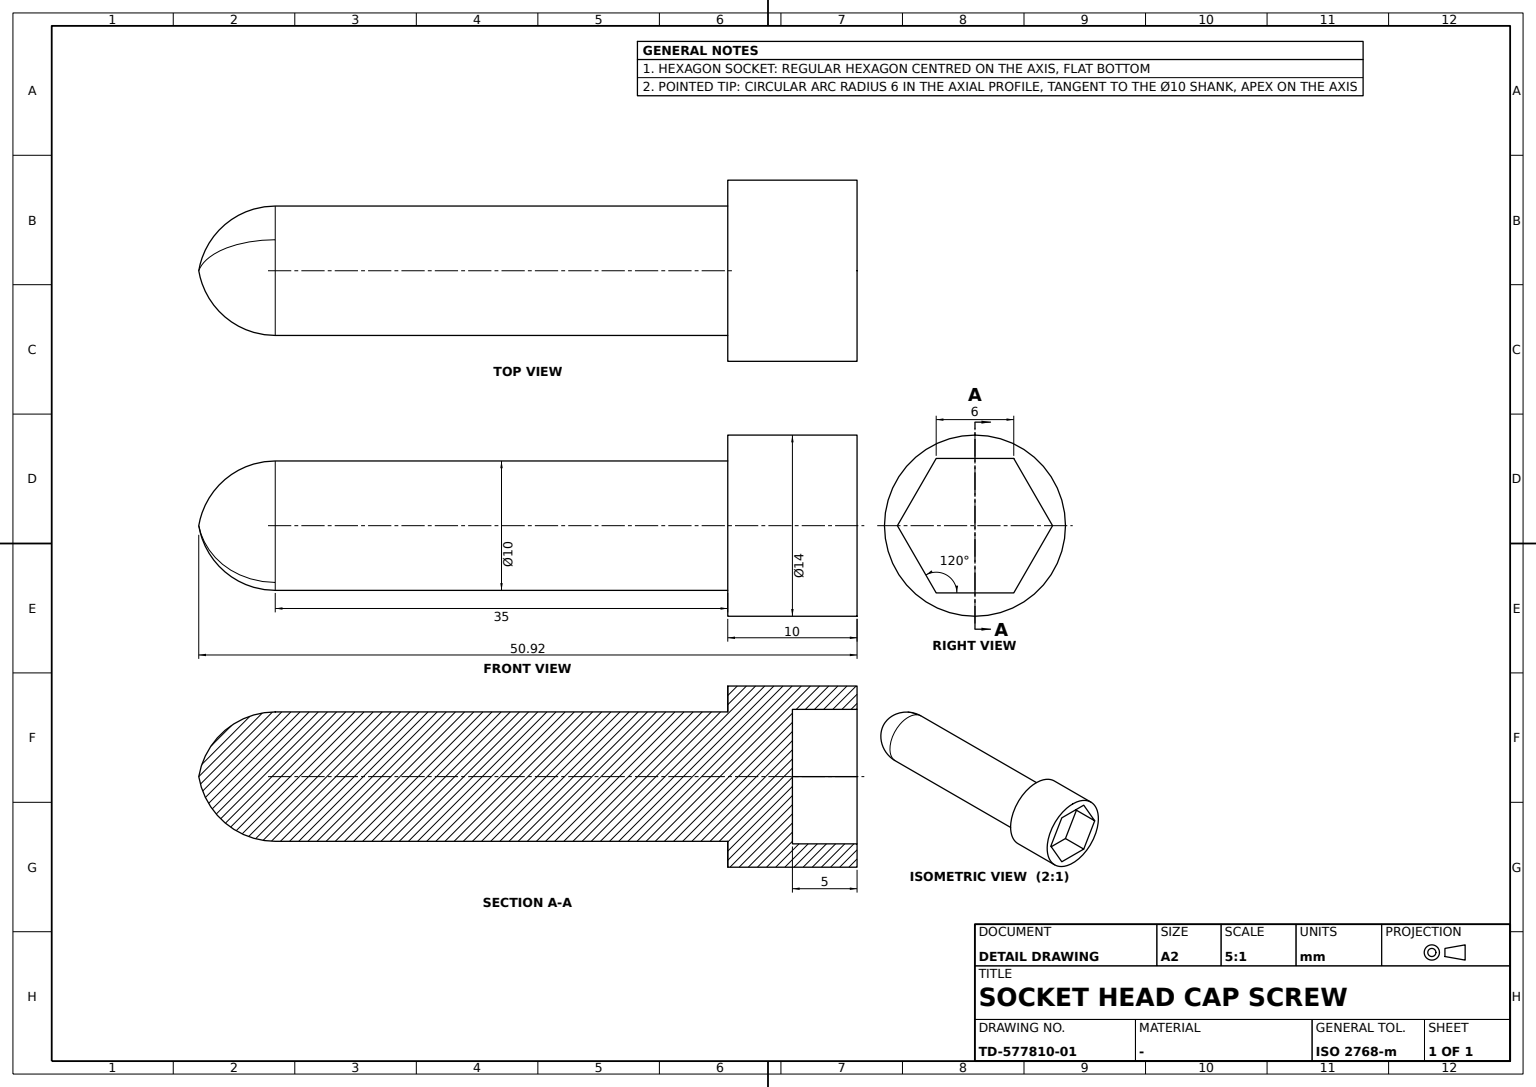
ISO-10303-21;
HEADER;
FILE_DESCRIPTION((''),'2;1');
FILE_NAME('','',(''),(''),'','','');
FILE_SCHEMA(('AUTOMOTIVE_DESIGN'));
ENDSEC;
DATA;
#1=APPLICATION_CONTEXT('');
#2=PRODUCT_CONTEXT('',#1,'mechanical');
#3=PRODUCT('','','',(#2));
#4=PRODUCT_DEFINITION_FORMATION('','',#3);
#5=PRODUCT_DEFINITION_CONTEXT('',#1,'design');
#6=PRODUCT_DEFINITION('','',#4,#5);
#7=PRODUCT_DEFINITION_SHAPE('','',#6);
#8=(LENGTH_UNIT()NAMED_UNIT(*)SI_UNIT(.MILLI.,.METRE.));
#9=(NAMED_UNIT(*)PLANE_ANGLE_UNIT()SI_UNIT($,.RADIAN.));
#10=(NAMED_UNIT(*)SI_UNIT($,.STERADIAN.)SOLID_ANGLE_UNIT());
#11=UNCERTAINTY_MEASURE_WITH_UNIT(LENGTH_MEASURE(0.005),#8,'distance_accuracy_value','');
#12=(GEOMETRIC_REPRESENTATION_CONTEXT(3)GLOBAL_UNCERTAINTY_ASSIGNED_CONTEXT((#11))GLOBAL_UNIT_ASSIGNED_CONTEXT((#8,#9,#10))REPRESENTATION_CONTEXT('',''));
#13=CARTESIAN_POINT('',(0.,-3.,-5.196152));
#14=VERTEX_POINT('',#13);
#15=CARTESIAN_POINT('',(0.,3.,-5.196152));
#16=VERTEX_POINT('',#15);
#17=CARTESIAN_POINT('',(0.,0.,-5.196152));
#18=DIRECTION('',(0.,1.,0.));
#19=VECTOR('',#18,1000.);
#20=LINE('',#17,#19);
#21=EDGE_CURVE('',#14,#16,#20,.T.);
#22=ORIENTED_EDGE('',*,*,#21,.T.);
#23=CARTESIAN_POINT('',(-5.,3.,-5.196152));
#24=VERTEX_POINT('',#23);
#25=DIRECTION('',(-1.,0.,0.));
#26=VECTOR('',#25,1000.);
#27=LINE('',#15,#26);
#28=EDGE_CURVE('',#16,#24,#27,.T.);
#29=ORIENTED_EDGE('',*,*,#28,.T.);
#30=CARTESIAN_POINT('',(-5.,-3.,-5.196152));
#31=VERTEX_POINT('',#30);
#32=LINE('',#30,#19);
#33=EDGE_CURVE('',#31,#24,#32,.T.);
#34=ORIENTED_EDGE('',*,*,#33,.F.);
#35=LINE('',#13,#26);
#36=EDGE_CURVE('',#14,#31,#35,.T.);
#37=ORIENTED_EDGE('',*,*,#36,.F.);
#38=EDGE_LOOP('',(#22,#29,#34,#37));
#39=FACE_BOUND('',#38,.T.);
#40=DIRECTION('',(0.,0.,1.));
#41=AXIS2_PLACEMENT_3D('',#13,#40,#18);
#42=PLANE('',#41);
#43=ADVANCED_FACE('',(#39),#42,.T.);
#44=CARTESIAN_POINT('',(-10.,0.,7.));
#45=VERTEX_POINT('',#44);
#46=CARTESIAN_POINT('',(-10.,0.,0.));
#47=AXIS2_PLACEMENT_3D('',#46,#25,#40);
#48=CIRCLE('',#47,7.);
#49=EDGE_CURVE('',#45,#45,#48,.T.);
#50=ORIENTED_EDGE('',*,*,#49,.F.);
#51=EDGE_LOOP('',(#50));
#52=FACE_BOUND('',#51,.T.);
#53=CARTESIAN_POINT('',(0.,0.,7.));
#54=VERTEX_POINT('',#53);
#55=CARTESIAN_POINT('',(0.,0.,0.));
#56=AXIS2_PLACEMENT_3D('',#55,#25,#40);
#57=CIRCLE('',#56,7.);
#58=EDGE_CURVE('',#54,#54,#57,.T.);
#59=ORIENTED_EDGE('',*,*,#58,.T.);
#60=EDGE_LOOP('',(#59));
#61=FACE_BOUND('',#60,.T.);
#62=CARTESIAN_POINT('',(-25.45804,0.,0.));
#63=AXIS2_PLACEMENT_3D('',#62,#25,#18);
#64=CYLINDRICAL_SURFACE('',#63,7.);
#65=ADVANCED_FACE('',(#52,#61),#64,.T.);
#66=CARTESIAN_POINT('',(-50.91608,0.,0.));
#67=VERTEX_POINT('',#66);
#68=CARTESIAN_POINT('',(-45.,-2.397128,-4.387913));
#69=VERTEX_POINT('',#68);
#70=CARTESIAN_POINT('',(-46.403166,-2.397,-4.38768));
#71=CARTESIAN_POINT('',(-49.203342,-1.904979,-3.487041));
#72=CARTESIAN_POINT('',(-50.681957,-0.663283,-1.214132));
#73=B_SPLINE_CURVE_WITH_KNOTS('',3,(#68,#70,#71,#72,#66),.UNSPECIFIED.,.F.,.F.,(4,1,4),(1.004688475,5.214733218,9.424777961),.UNSPECIFIED.);
#74=EDGE_CURVE('',#67,#69,#73,.F.);
#75=ORIENTED_EDGE('',*,*,#74,.F.);
#76=CARTESIAN_POINT('',(-45.,2.397128,4.387913));
#77=VERTEX_POINT('',#76);
#78=CARTESIAN_POINT('',(-50.681957,0.663283,1.214132));
#79=CARTESIAN_POINT('',(-49.203342,1.904979,3.487041));
#80=CARTESIAN_POINT('',(-46.403166,2.397,4.38768));
#81=B_SPLINE_CURVE_WITH_KNOTS('',3,(#66,#78,#79,#80,#76),.UNSPECIFIED.,.F.,.F.,(4,1,4),(1.004688475,5.214733218,9.424777961),.UNSPECIFIED.);
#82=EDGE_CURVE('',#67,#77,#81,.T.);
#83=ORIENTED_EDGE('',*,*,#82,.T.);
#84=CARTESIAN_POINT('',(-45.,-1.248375,-5.015479));
#85=CARTESIAN_POINT('',(-45.,1.558696,-5.316123));
#86=CARTESIAN_POINT('',(-45.,4.863313,-2.65684));
#87=CARTESIAN_POINT('',(-45.,5.31553,1.560716));
#88=CARTESIAN_POINT('',(-45.,3.545881,3.760346));
#89=B_SPLINE_CURVE_WITH_KNOTS('',3,(#68,#84,#85,#86,#87,#88,#76),.UNSPECIFIED.,.F.,.F.,(4,1,1,1,4),(26.061944902,29.988935719,33.915926536,37.842917353,41.76990817),.UNSPECIFIED.);
#90=EDGE_CURVE('',#77,#69,#89,.F.);
#91=ORIENTED_EDGE('',*,*,#90,.T.);
#92=EDGE_LOOP('',(#75,#83,#91));
#93=FACE_BOUND('',#92,.T.);
#94=CARTESIAN_POINT('',(-50.635133,0.79594,1.456959));
#95=CARTESIAN_POINT('',(-50.635133,1.253413,1.206799));
#96=CARTESIAN_POINT('',(-50.635133,1.614202,0.777583));
#97=CARTESIAN_POINT('',(-50.635133,1.777866,0.217642));
#98=CARTESIAN_POINT('',(-50.635133,1.636262,-0.893894));
#99=CARTESIAN_POINT('',(-50.635133,0.777445,-1.613615));
#100=CARTESIAN_POINT('',(-50.635133,0.217843,-1.778434));
#101=CARTESIAN_POINT('',(-50.635133,-0.338265,-1.706747));
#102=CARTESIAN_POINT('',(-50.635133,-0.79594,-1.456959));
#103=CARTESIAN_POINT('',(-49.77342,1.545475,2.828972));
#104=CARTESIAN_POINT('',(-49.77342,2.433747,2.343238));
#105=CARTESIAN_POINT('',(-49.77342,3.13429,1.509831));
#106=CARTESIAN_POINT('',(-49.77342,3.452077,0.422595));
#107=CARTESIAN_POINT('',(-49.77342,3.177124,-1.735671));
#108=CARTESIAN_POINT('',(-49.77342,1.509563,-3.133152));
#109=CARTESIAN_POINT('',(-49.77342,0.422986,-3.453179));
#110=CARTESIAN_POINT('',(-49.77342,-0.656807,-3.313985));
#111=CARTESIAN_POINT('',(-49.77342,-1.545475,-2.828972));
#112=CARTESIAN_POINT('',(-48.368952,2.114549,3.870656));
#113=CARTESIAN_POINT('',(-48.368952,3.329901,3.206064));
#114=CARTESIAN_POINT('',(-48.368952,4.288398,2.06578));
#115=CARTESIAN_POINT('',(-48.368952,4.7232,0.578203));
#116=CARTESIAN_POINT('',(-48.368952,4.347004,-2.374779));
#117=CARTESIAN_POINT('',(-48.368952,2.065414,-4.28684));
#118=CARTESIAN_POINT('',(-48.368952,0.578737,-4.724708));
#119=CARTESIAN_POINT('',(-48.368952,-0.898657,-4.534259));
#120=CARTESIAN_POINT('',(-48.368952,-2.114549,-3.870656));
#121=CARTESIAN_POINT('',(-46.683799,2.396975,4.387633));
#122=CARTESIAN_POINT('',(-46.683799,3.774654,3.634277));
#123=CARTESIAN_POINT('',(-46.683799,4.86117,2.341693));
#124=CARTESIAN_POINT('',(-46.683799,5.354046,0.65543));
#125=CARTESIAN_POINT('',(-46.683799,4.927605,-2.691963));
#126=CARTESIAN_POINT('',(-46.683799,2.341278,-4.859405));
#127=CARTESIAN_POINT('',(-46.683799,0.656035,-5.355756));
#128=CARTESIAN_POINT('',(-46.683799,-1.018685,-5.13987));
#129=CARTESIAN_POINT('',(-46.683799,-2.396975,-4.387633));
#130=CARTESIAN_POINT('',(-45.,3.774894,3.634509));
#131=CARTESIAN_POINT('',(-45.,4.86148,2.341842));
#132=CARTESIAN_POINT('',(-45.,5.354387,0.655472));
#133=CARTESIAN_POINT('',(-45.,4.927918,-2.692134));
#134=CARTESIAN_POINT('',(-45.,2.341427,-4.859715));
#135=CARTESIAN_POINT('',(-45.,0.656077,-5.356097));
#136=CARTESIAN_POINT('',(-45.,-1.018749,-5.140197));
#137=B_SPLINE_SURFACE_WITH_KNOTS('',5,5,((#66,#66,#66,#66,#66,#66,#66,#66,#66),(#94,#95,#96,#97,#98,#99,#100,#101,#102),(#103,#104,#105,#106,#107,#108,#109,#110,#111),(#112,#113,#114,#115,#116,#117,#118,#119,#120),(#121,#122,#123,#124,#125,#126,#127,#128,#129),(#76,#130,#131,#132,#133,#134,#135,#136,#68)),.UNSPECIFIED.,.F.,.F.,.F.,(6,6),(6,3,6),(0.,0.045),(0.,0.0055,0.011),.UNSPECIFIED.);
#138=ADVANCED_FACE('',(#93),#137,.T.);
#139=CARTESIAN_POINT('',(0.,-6.,0.));
#140=VERTEX_POINT('',#139);
#141=CARTESIAN_POINT('',(0.,-4.5,-2.598076));
#142=DIRECTION('',(0.,0.5,-0.866025404));
#143=VECTOR('',#142,1000.);
#144=LINE('',#141,#143);
#145=EDGE_CURVE('',#140,#14,#144,.T.);
#146=ORIENTED_EDGE('',*,*,#145,.T.);
#147=ORIENTED_EDGE('',*,*,#36,.T.);
#148=CARTESIAN_POINT('',(-5.,-6.,0.));
#149=VERTEX_POINT('',#148);
#150=LINE('',#148,#143);
#151=EDGE_CURVE('',#149,#31,#150,.T.);
#152=ORIENTED_EDGE('',*,*,#151,.F.);
#153=LINE('',#139,#26);
#154=EDGE_CURVE('',#140,#149,#153,.T.);
#155=ORIENTED_EDGE('',*,*,#154,.F.);
#156=EDGE_LOOP('',(#146,#147,#152,#155));
#157=FACE_BOUND('',#156,.T.);
#158=DIRECTION('',(0.,0.866025404,0.5));
#159=AXIS2_PLACEMENT_3D('',#139,#158,#142);
#160=PLANE('',#159);
#161=ADVANCED_FACE('',(#157),#160,.T.);
#162=ORIENTED_EDGE('',*,*,#154,.T.);
#163=CARTESIAN_POINT('',(-5.,-3.,5.196152));
#164=VERTEX_POINT('',#163);
#165=DIRECTION('',(0.,-0.5,-0.866025404));
#166=VECTOR('',#165,1000.);
#167=LINE('',#163,#166);
#168=EDGE_CURVE('',#164,#149,#167,.T.);
#169=ORIENTED_EDGE('',*,*,#168,.F.);
#170=CARTESIAN_POINT('',(0.,-3.,5.196152));
#171=VERTEX_POINT('',#170);
#172=LINE('',#170,#26);
#173=EDGE_CURVE('',#171,#164,#172,.T.);
#174=ORIENTED_EDGE('',*,*,#173,.F.);
#175=CARTESIAN_POINT('',(0.,-4.5,2.598076));
#176=LINE('',#175,#166);
#177=EDGE_CURVE('',#171,#140,#176,.T.);
#178=ORIENTED_EDGE('',*,*,#177,.T.);
#179=EDGE_LOOP('',(#162,#169,#174,#178));
#180=FACE_BOUND('',#179,.T.);
#181=DIRECTION('',(0.,0.866025404,-0.5));
#182=AXIS2_PLACEMENT_3D('',#170,#181,#165);
#183=PLANE('',#182);
#184=ADVANCED_FACE('',(#180),#183,.T.);
#185=CARTESIAN_POINT('',(-10.,0.,5.));
#186=VERTEX_POINT('',#185);
#187=CIRCLE('',#47,5.);
#188=EDGE_CURVE('',#186,#186,#187,.T.);
#189=ORIENTED_EDGE('',*,*,#188,.T.);
#190=EDGE_LOOP('',(#189));
#191=FACE_BOUND('',#190,.T.);
#192=ORIENTED_EDGE('',*,*,#90,.F.);
#193=CARTESIAN_POINT('',(-45.,1.248375,5.015479));
#194=CARTESIAN_POINT('',(-45.,-1.558696,5.316123));
#195=CARTESIAN_POINT('',(-45.,-4.863313,2.65684));
#196=CARTESIAN_POINT('',(-45.,-5.31553,-1.560716));
#197=CARTESIAN_POINT('',(-45.,-3.545881,-3.760346));
#198=B_SPLINE_CURVE_WITH_KNOTS('',3,(#76,#193,#194,#195,#196,#197,#68),.UNSPECIFIED.,.F.,.F.,(4,1,1,1,4),(41.76990817,45.696898987,49.623889804,53.550880621,57.477871438),.UNSPECIFIED.);
#199=EDGE_CURVE('',#69,#77,#198,.F.);
#200=ORIENTED_EDGE('',*,*,#199,.F.);
#201=EDGE_LOOP('',(#192,#200));
#202=FACE_BOUND('',#201,.T.);
#203=CYLINDRICAL_SURFACE('',#63,5.);
#204=ADVANCED_FACE('',(#191,#202),#203,.T.);
#205=ORIENTED_EDGE('',*,*,#49,.T.);
#206=EDGE_LOOP('',(#205));
#207=FACE_BOUND('',#206,.T.);
#208=ORIENTED_EDGE('',*,*,#188,.F.);
#209=EDGE_LOOP('',(#208));
#210=FACE_BOUND('',#209,.T.);
#211=AXIS2_PLACEMENT_3D('',#44,#25,#18);
#212=PLANE('',#211);
#213=ADVANCED_FACE('',(#207,#210),#212,.T.);
#214=ORIENTED_EDGE('',*,*,#151,.T.);
#215=ORIENTED_EDGE('',*,*,#33,.T.);
#216=CARTESIAN_POINT('',(-5.,6.,0.));
#217=VERTEX_POINT('',#216);
#218=DIRECTION('',(0.,0.5,0.866025404));
#219=VECTOR('',#218,1000.);
#220=LINE('',#23,#219);
#221=EDGE_CURVE('',#24,#217,#220,.T.);
#222=ORIENTED_EDGE('',*,*,#221,.T.);
#223=CARTESIAN_POINT('',(-5.,3.,5.196152));
#224=VERTEX_POINT('',#223);
#225=DIRECTION('',(0.,-0.5,0.866025404));
#226=VECTOR('',#225,1000.);
#227=LINE('',#216,#226);
#228=EDGE_CURVE('',#217,#224,#227,.T.);
#229=ORIENTED_EDGE('',*,*,#228,.T.);
#230=DIRECTION('',(0.,-1.,0.));
#231=VECTOR('',#230,1000.);
#232=LINE('',#223,#231);
#233=EDGE_CURVE('',#224,#164,#232,.T.);
#234=ORIENTED_EDGE('',*,*,#233,.T.);
#235=ORIENTED_EDGE('',*,*,#168,.T.);
#236=EDGE_LOOP('',(#214,#215,#222,#229,#234,#235));
#237=FACE_BOUND('',#236,.T.);
#238=CARTESIAN_POINT('',(-5.,0.,0.));
#239=DIRECTION('',(1.,0.,0.));
#240=AXIS2_PLACEMENT_3D('',#238,#239,#18);
#241=PLANE('',#240);
#242=ADVANCED_FACE('',(#237),#241,.T.);
#243=ORIENTED_EDGE('',*,*,#145,.F.);
#244=ORIENTED_EDGE('',*,*,#177,.F.);
#245=CARTESIAN_POINT('',(0.,3.,5.196152));
#246=VERTEX_POINT('',#245);
#247=CARTESIAN_POINT('',(0.,0.,5.196152));
#248=LINE('',#247,#231);
#249=EDGE_CURVE('',#246,#171,#248,.T.);
#250=ORIENTED_EDGE('',*,*,#249,.F.);
#251=CARTESIAN_POINT('',(0.,6.,0.));
#252=VERTEX_POINT('',#251);
#253=CARTESIAN_POINT('',(0.,4.5,2.598076));
#254=LINE('',#253,#226);
#255=EDGE_CURVE('',#252,#246,#254,.T.);
#256=ORIENTED_EDGE('',*,*,#255,.F.);
#257=CARTESIAN_POINT('',(0.,4.5,-2.598076));
#258=LINE('',#257,#219);
#259=EDGE_CURVE('',#16,#252,#258,.T.);
#260=ORIENTED_EDGE('',*,*,#259,.F.);
#261=ORIENTED_EDGE('',*,*,#21,.F.);
#262=EDGE_LOOP('',(#243,#244,#250,#256,#260,#261));
#263=FACE_BOUND('',#262,.T.);
#264=ORIENTED_EDGE('',*,*,#58,.F.);
#265=EDGE_LOOP('',(#264));
#266=FACE_BOUND('',#265,.T.);
#267=AXIS2_PLACEMENT_3D('',#55,#25,#18);
#268=PLANE('',#267);
#269=ADVANCED_FACE('',(#263,#266),#268,.F.);
#270=ORIENTED_EDGE('',*,*,#199,.T.);
#271=ORIENTED_EDGE('',*,*,#82,.F.);
#272=ORIENTED_EDGE('',*,*,#74,.T.);
#273=EDGE_LOOP('',(#270,#271,#272));
#274=FACE_BOUND('',#273,.T.);
#275=CARTESIAN_POINT('',(-50.635133,-1.101067,-1.290243));
#276=CARTESIAN_POINT('',(-50.635133,-1.362663,-1.04373));
#277=CARTESIAN_POINT('',(-50.635133,-1.552372,-0.732268));
#278=CARTESIAN_POINT('',(-50.635133,-1.750681,-0.041324));
#279=CARTESIAN_POINT('',(-50.635133,-1.5852,0.658217));
#280=CARTESIAN_POINT('',(-50.635133,-1.410358,0.978263));
#281=CARTESIAN_POINT('',(-50.635133,-0.911124,1.495475));
#282=CARTESIAN_POINT('',(-50.635133,-0.222568,1.701922));
#283=CARTESIAN_POINT('',(-50.635133,0.142018,1.710571));
#284=CARTESIAN_POINT('',(-50.635133,0.490793,1.623637));
#285=CARTESIAN_POINT('',(-49.77342,-2.137938,-2.505261));
#286=CARTESIAN_POINT('',(-49.77342,-2.645878,-2.026607));
#287=CARTESIAN_POINT('',(-49.77342,-3.014236,-1.421843));
#288=CARTESIAN_POINT('',(-49.77342,-3.399292,-0.08024));
#289=CARTESIAN_POINT('',(-49.77342,-3.077977,1.278059));
#290=CARTESIAN_POINT('',(-49.77342,-2.738487,1.899491));
#291=CARTESIAN_POINT('',(-49.77342,-1.769126,2.903759));
#292=CARTESIAN_POINT('',(-49.77342,-0.432159,3.304617));
#293=CARTESIAN_POINT('',(-49.77342,0.275756,3.32141));
#294=CARTESIAN_POINT('',(-49.77342,0.952972,3.152611));
#295=CARTESIAN_POINT('',(-48.368952,-2.925169,-3.427748));
#296=CARTESIAN_POINT('',(-48.368952,-3.620143,-2.772843));
#297=CARTESIAN_POINT('',(-48.368952,-4.124137,-1.945393));
#298=CARTESIAN_POINT('',(-48.368952,-4.650978,-0.109785));
#299=CARTESIAN_POINT('',(-48.368952,-4.211349,1.748665));
#300=CARTESIAN_POINT('',(-48.368952,-3.746853,2.598921));
#301=CARTESIAN_POINT('',(-48.368952,-2.420553,3.97298));
#302=CARTESIAN_POINT('',(-48.368952,-0.591288,4.521442));
#303=CARTESIAN_POINT('',(-48.368952,0.377295,4.544419));
#304=CARTESIAN_POINT('',(-48.368952,1.303875,4.313465));
#305=CARTESIAN_POINT('',(-46.683799,-3.315865,-3.88557));
#306=CARTESIAN_POINT('',(-46.683799,-4.103662,-3.143193));
#307=CARTESIAN_POINT('',(-46.683799,-4.67497,-2.205227));
#308=CARTESIAN_POINT('',(-46.683799,-5.272178,-0.124449));
#309=CARTESIAN_POINT('',(-46.683799,-4.773831,1.982223));
#310=CARTESIAN_POINT('',(-46.683799,-4.247295,2.946041));
#311=CARTESIAN_POINT('',(-46.683799,-2.74385,4.503625));
#312=CARTESIAN_POINT('',(-46.683799,-0.670263,5.125341));
#313=CARTESIAN_POINT('',(-46.683799,0.427688,5.151387));
#314=CARTESIAN_POINT('',(-46.683799,1.478025,4.889586));
#315=CARTESIAN_POINT('',(-45.,-3.316076,-3.885817));
#316=CARTESIAN_POINT('',(-45.,-4.103923,-3.143394));
#317=CARTESIAN_POINT('',(-45.,-4.675268,-2.205367));
#318=CARTESIAN_POINT('',(-45.,-5.272514,-0.124457));
#319=CARTESIAN_POINT('',(-45.,-4.774135,1.982349));
#320=CARTESIAN_POINT('',(-45.,-4.247565,2.946229));
#321=CARTESIAN_POINT('',(-45.,-2.744025,4.503912));
#322=CARTESIAN_POINT('',(-45.,-0.670306,5.125667));
#323=CARTESIAN_POINT('',(-45.,0.427716,5.151715));
#324=CARTESIAN_POINT('',(-45.,1.478119,4.889898));
#325=B_SPLINE_SURFACE_WITH_KNOTS('',5,5,((#66,#66,#66,#66,#66,#66,#66,#66,#66,#66,#66,#66),(#102,#275,#276,#277,#278,#279,#280,#281,#282,#283,#284,#94),(#111,#285,#286,#287,#288,#289,#290,#291,#292,#293,#294,#103),(#120,#295,#296,#297,#298,#299,#300,#301,#302,#303,#304,#112),(#129,#305,#306,#307,#308,#309,#310,#311,#312,#313,#314,#121),(#68,#315,#316,#317,#318,#319,#320,#321,#322,#323,#324,#76)),.UNSPECIFIED.,.F.,.F.,.F.,(6,6),(6,3,3,6),(0.,0.045),(0.,0.003666667,0.007333333,0.011),.UNSPECIFIED.);
#326=ADVANCED_FACE('',(#274),#325,.T.);
#327=LINE('',#251,#26);
#328=EDGE_CURVE('',#252,#217,#327,.T.);
#329=ORIENTED_EDGE('',*,*,#328,.T.);
#330=ORIENTED_EDGE('',*,*,#221,.F.);
#331=ORIENTED_EDGE('',*,*,#28,.F.);
#332=ORIENTED_EDGE('',*,*,#259,.T.);
#333=EDGE_LOOP('',(#329,#330,#331,#332));
#334=FACE_BOUND('',#333,.T.);
#335=DIRECTION('',(0.,-0.866025404,0.5));
#336=AXIS2_PLACEMENT_3D('',#15,#335,#218);
#337=PLANE('',#336);
#338=ADVANCED_FACE('',(#334),#337,.T.);
#339=ORIENTED_EDGE('',*,*,#255,.T.);
#340=LINE('',#245,#26);
#341=EDGE_CURVE('',#246,#224,#340,.T.);
#342=ORIENTED_EDGE('',*,*,#341,.T.);
#343=ORIENTED_EDGE('',*,*,#228,.F.);
#344=ORIENTED_EDGE('',*,*,#328,.F.);
#345=EDGE_LOOP('',(#339,#342,#343,#344));
#346=FACE_BOUND('',#345,.T.);
#347=DIRECTION('',(0.,-0.866025404,-0.5));
#348=AXIS2_PLACEMENT_3D('',#251,#347,#225);
#349=PLANE('',#348);
#350=ADVANCED_FACE('',(#346),#349,.T.);
#351=ORIENTED_EDGE('',*,*,#173,.T.);
#352=ORIENTED_EDGE('',*,*,#233,.F.);
#353=ORIENTED_EDGE('',*,*,#341,.F.);
#354=ORIENTED_EDGE('',*,*,#249,.T.);
#355=EDGE_LOOP('',(#351,#352,#353,#354));
#356=FACE_BOUND('',#355,.T.);
#357=DIRECTION('',(0.,0.,-1.));
#358=AXIS2_PLACEMENT_3D('',#245,#357,#230);
#359=PLANE('',#358);
#360=ADVANCED_FACE('',(#356),#359,.T.);
#361=CLOSED_SHELL('',(#43,#65,#138,#161,#184,#204,#213,#242,#269,#326,#338,#350,#360));
#362=MANIFOLD_SOLID_BREP('',#361);
#363=ADVANCED_BREP_SHAPE_REPRESENTATION('',(#362),#12);
#364=SHAPE_DEFINITION_REPRESENTATION(#7,#363);
ENDSEC;
END-ISO-10303-21;
